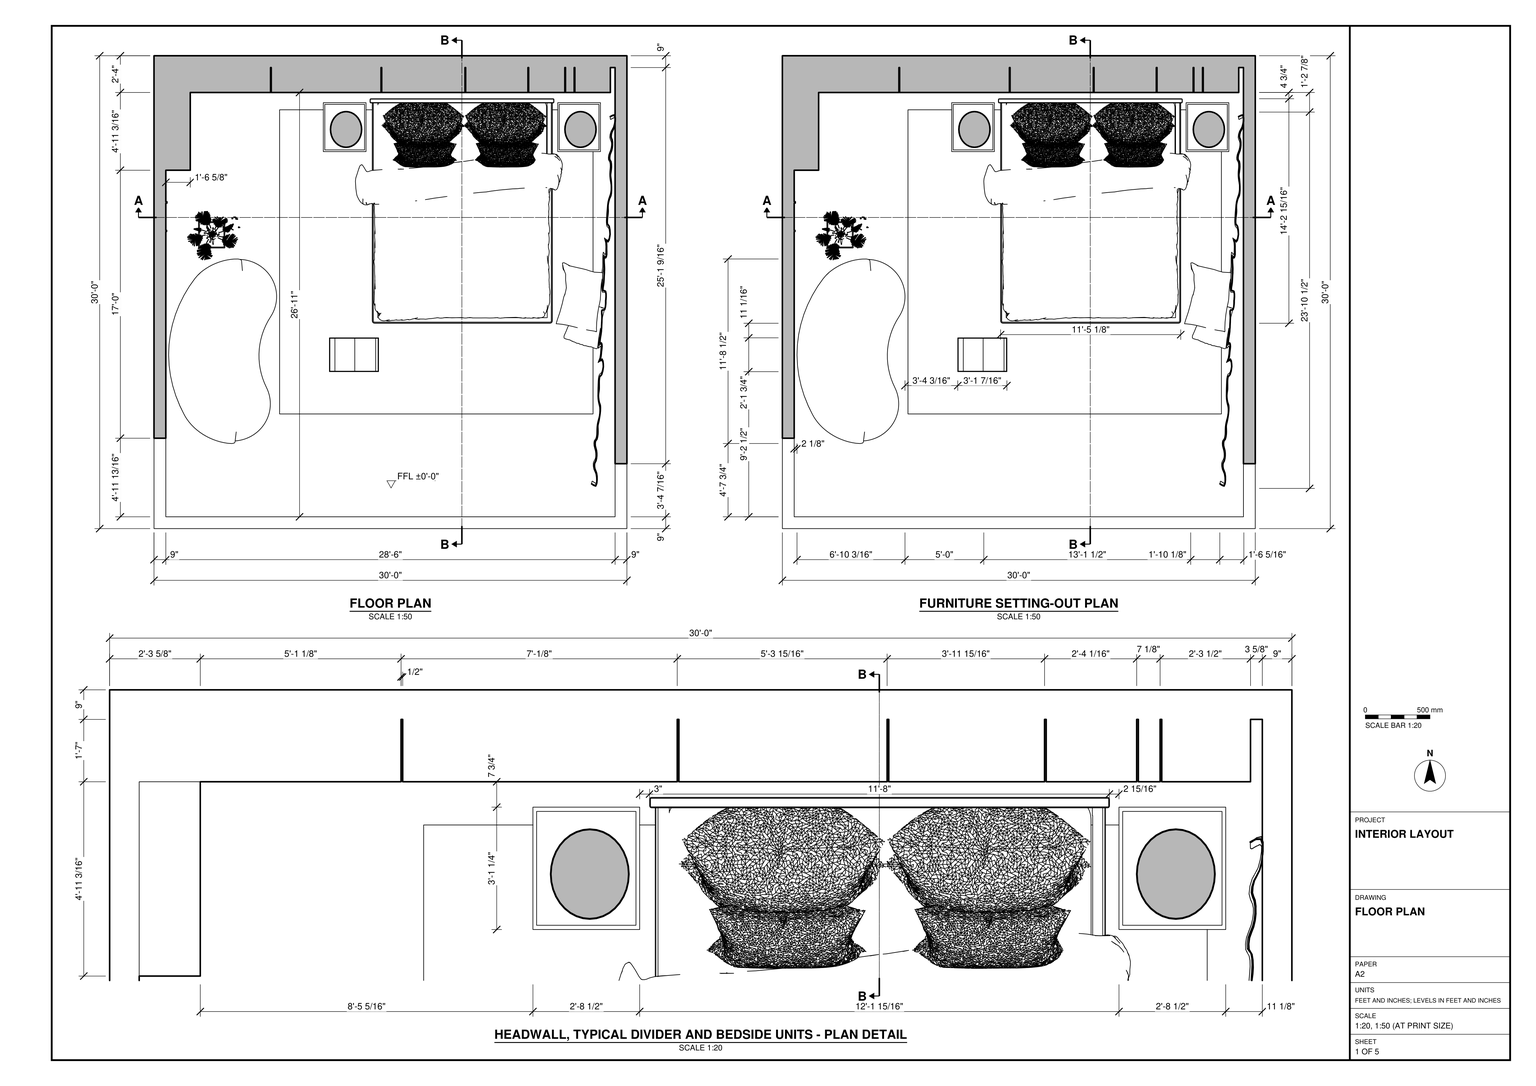
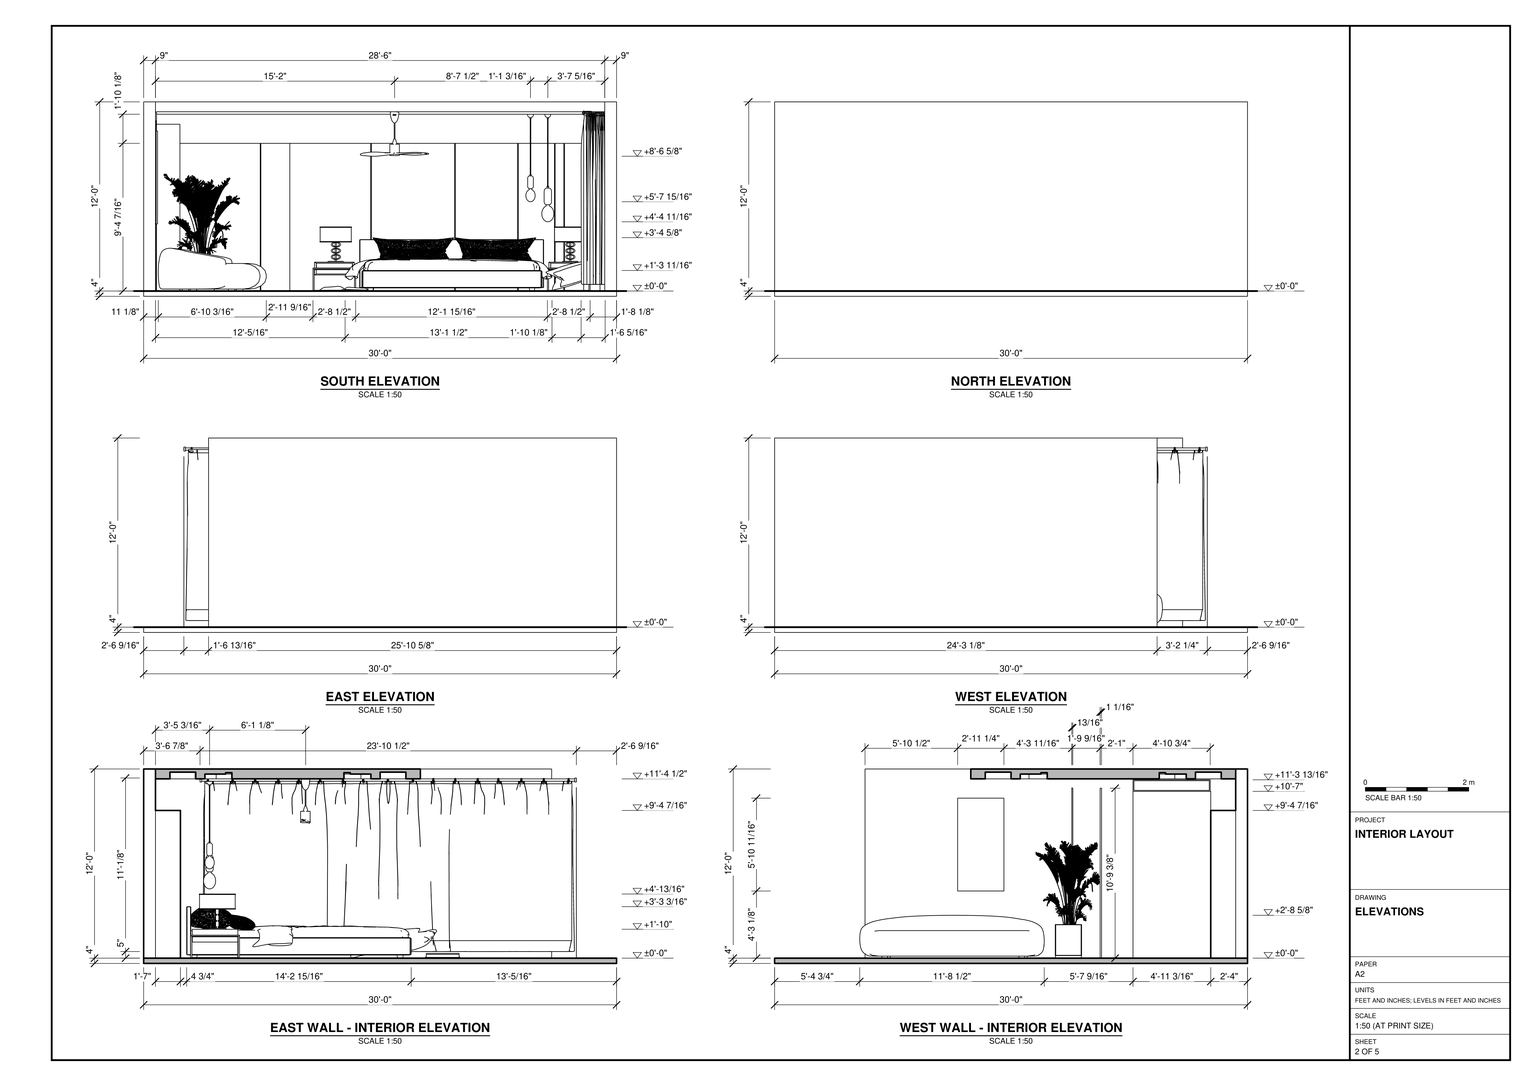
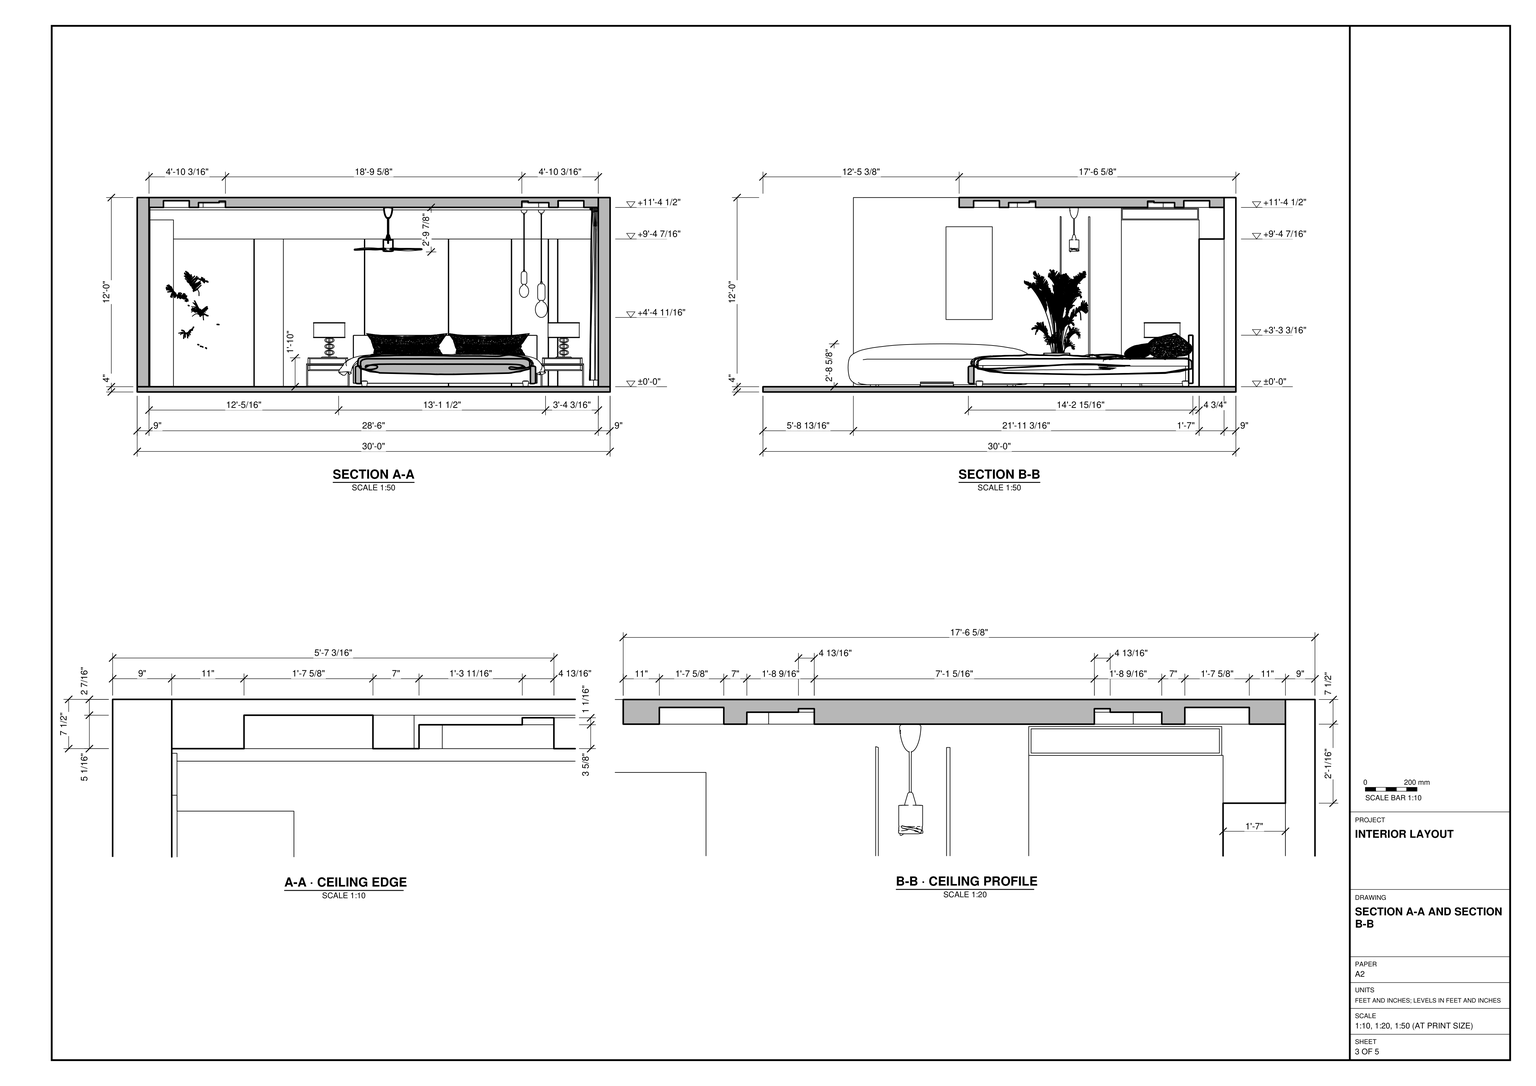
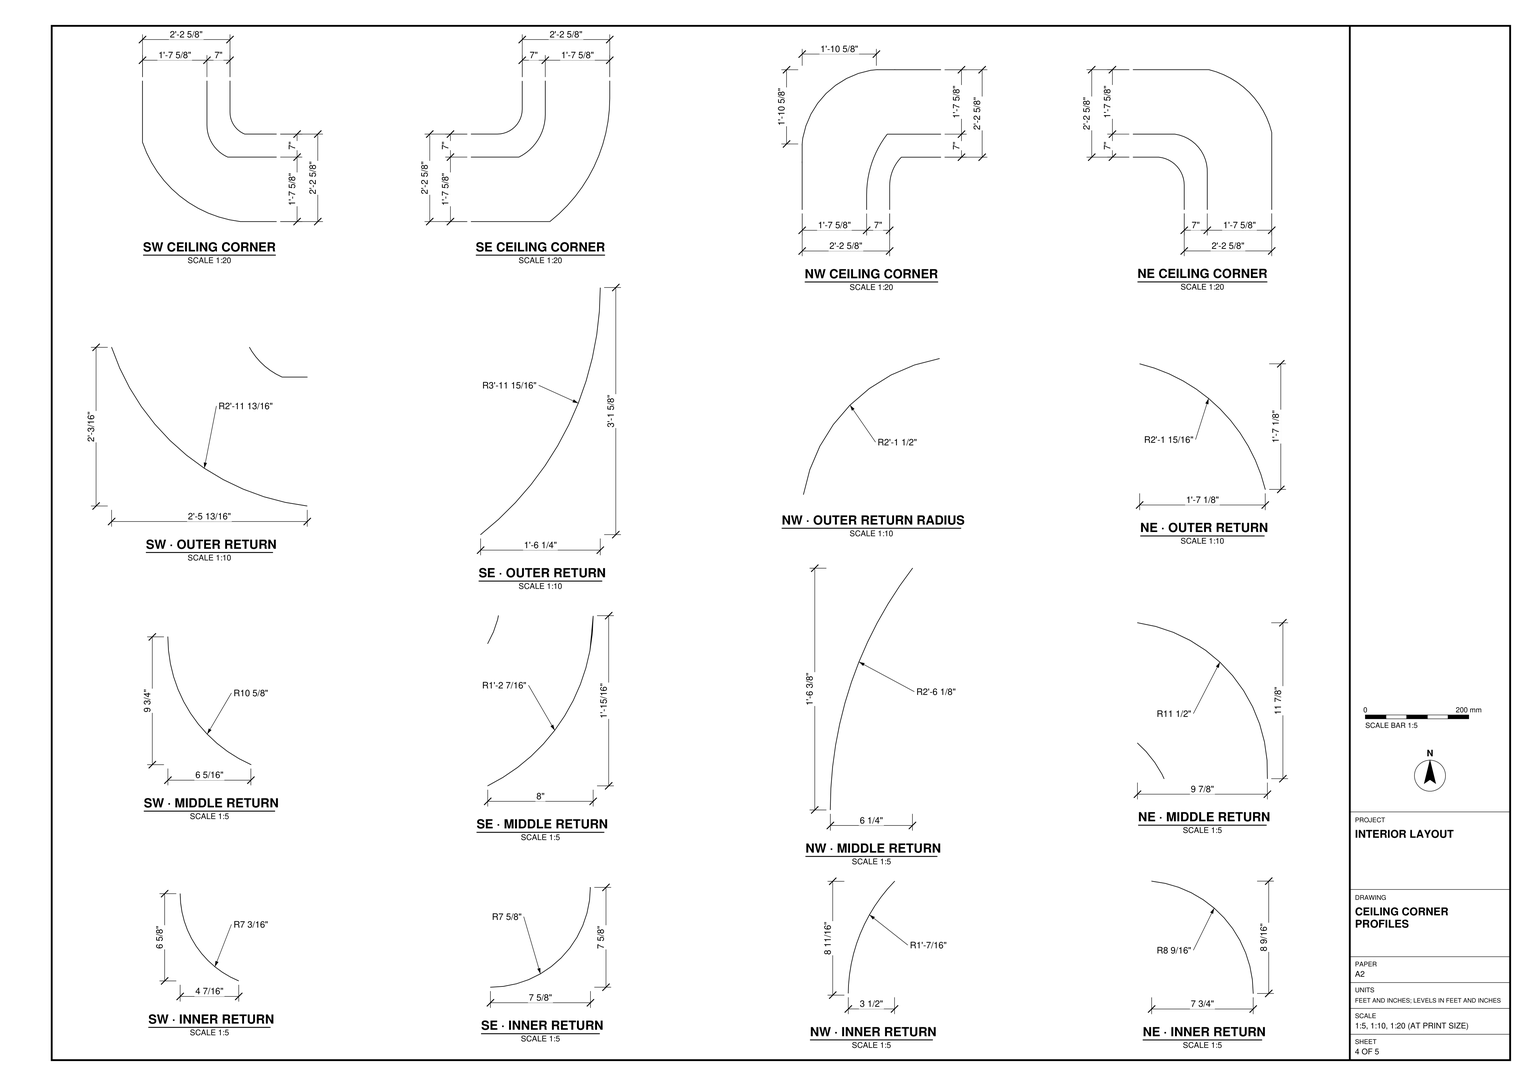
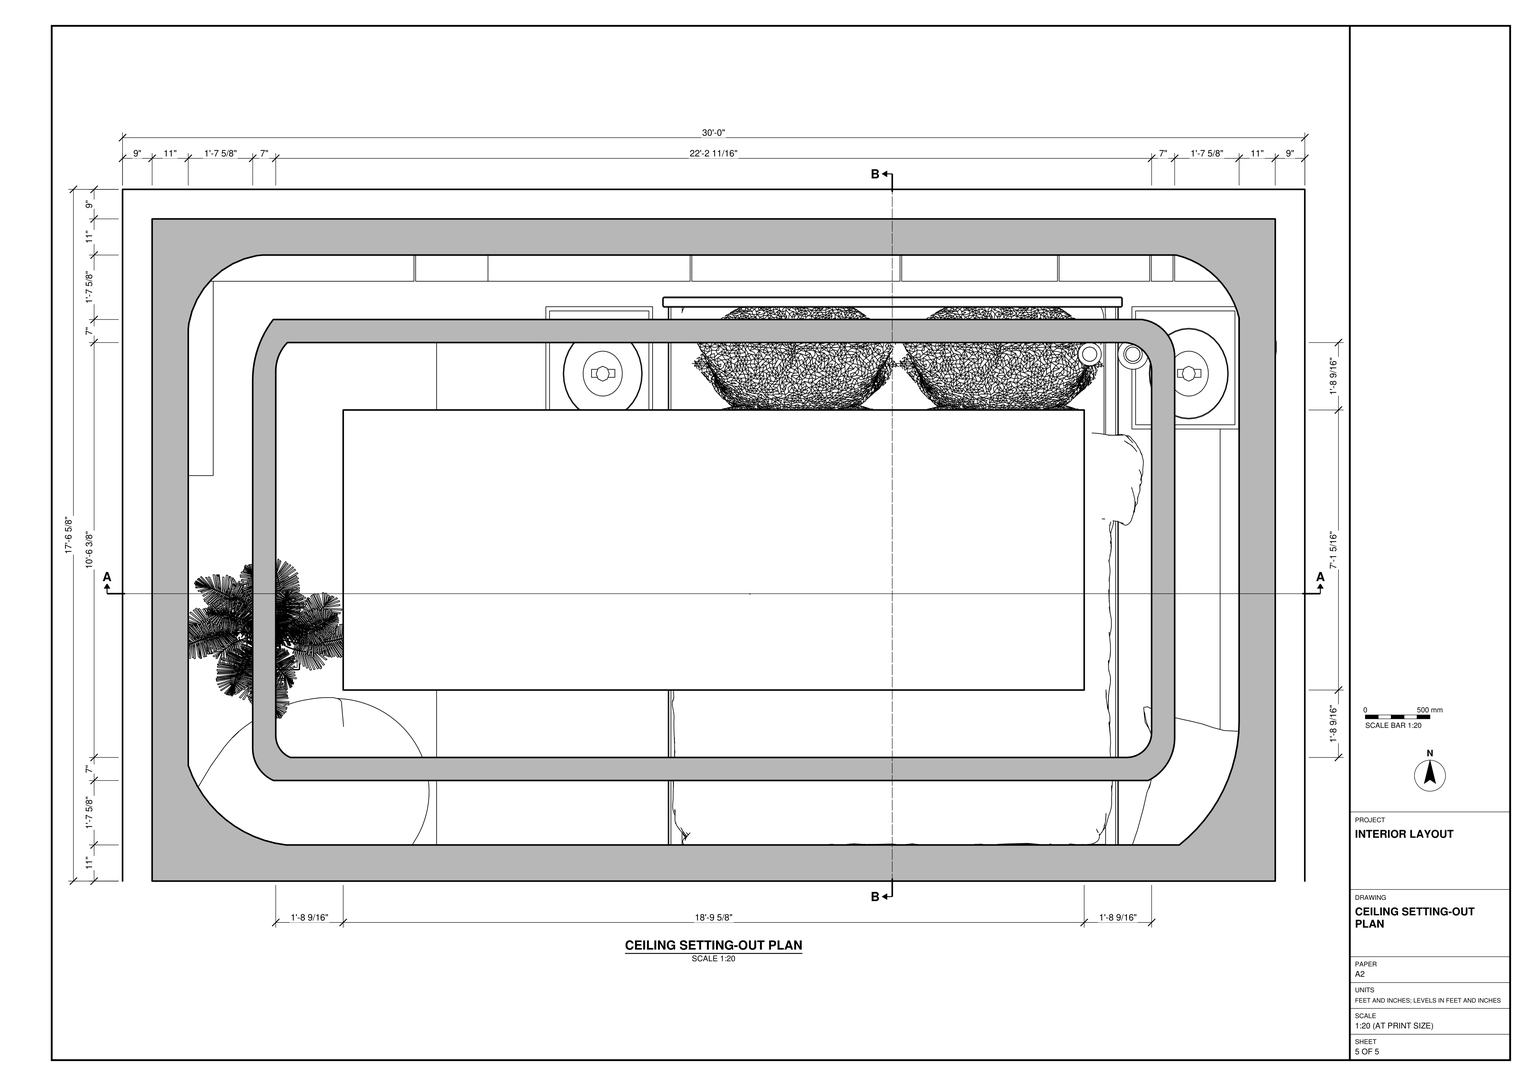
Build the bedroom interior in SketchUp from task_files/diagram_01.pdf. Work in feet and inches. The model is 30'-0" wide by 30'-0" deep and 12'-4" high overall, with one finished floor level at ±0'-0". Use the top of the 4" floor slab as the finished floor. Model the 9" walls along the north, east and west sides. Keep the south side open and stop each side wall where the floor plan shows it.

Build the headwall along the north wall, including its return, vertical panel divisions and the horizontal section above the panels. Use the sections and enlarged ceiling details to form the stepped recesses over the bed. Place the bed toward the east side of the headwall, with its foot facing south and a bedside unit on either side. Use the furniture setting-out plan for the bed footprint and the position of the curved sofa along the west side. Include the curtain along the east side, the ceiling fan, the lights and the plant in their drawn positions. Decor and loose items may be any suitable library components.

Keep the slab, walls and ceiling as separate groups or components. Do the same for each furniture or joinery piece, and use components for repeated parts. Save one SketchUp model as output_files/bedroom_with_panelled_headwall_and_stepped_ceiling.skp.

# SketchUp Ruby script. Lengths in inches.
U = 1.inch
M = Sketchup.active_model
def pt(a) = Geom::Point3d.new(a.map { |v| v * U })
def face(e, loops, mat)
  f = e.add_face(loops[0].map { |a| pt(a) })
  loops[1..].each { |l| e.add_face(l.map { |a| pt(a) }).erase! }
  f.material = f.back_material = mat if mat
  f
end
# faces: each face lists its corners as indices into pts; further lists are holes
def faces(e, pts, list, mat = nil) = list.each { |f| face(e, (f[0].is_a?(Array) ? f : [f]).map { |l| l.map { |i| pts[i] } }, mat) }
# xy, xz, yz: faces in a plane at the given z, y or x. An outline is a flat list of corners, or four numbers for a rectangle; further outlines are holes
def ring(l) = l.size == 4 ? [[l[0], l[1]], [l[2], l[1]], [l[2], l[3]], [l[0], l[3]]] : l.each_slice(2).to_a
def flat(e, list, mat, &to3) = list.each { |f| face(e, (f[0].is_a?(Array) ? f : [f]).map { |l| ring(l).map { |u, v| to3.(u, v) } }, mat) }
def xy(e, z, list, mat = nil) = flat(e, list, mat) { |x, y| [x, y, z] }
def xz(e, y, list, mat = nil) = flat(e, list, mat) { |x, z| [x, y, z] }
def yz(e, x, list, mat = nil) = flat(e, list, mat) { |y, z| [x, y, z] }
def lines(e, pts, list) = list.each { |a, b| e.add_line(pt(pts[a]), pt(pts[b])) }
# prism: a flat outline (further loops are holes) pulled along v
def prism(e, loops, v, mat = nil)
  f = face(e, loops, mat); d = Geom::Vector3d.new(v.map { |x| x * U })
  f.pushpull(f.normal.samedirection?(d) ? d.length : -d.length)
end
def box(e, o, s, mat = nil) = prism(e, [[o, [o[0] + s[0], o[1], o[2]], [o[0] + s[0], o[1] + s[1], o[2]], [o[0], o[1] + s[1], o[2]]]], [0, 0, s[2]], mat)
def at(x, y, z, deg = 0) = Geom::Transformation.translation(pt([x, y, z])) * Geom::Transformation.rotation(ORIGIN, Z_AXIS, deg.degrees)
def axes(o, x, y, z) = Geom::Transformation.new([*x, 0, *y, 0, *z, 0, *pt(o).to_a, 1])
def part(name) = M.definitions.add(name)
# library, detail: a bought-in or finely detailed component or shape, given as its bounding box
def library(name, o, s) = part(name).tap { |d| box(d.entities, o, s) }
def detail(e, o, s) = box(e.add_group.entities, o, s)
def put(e, d, t, mat = nil) = e.add_instance(d, t).tap { |i| i.material = mat if mat }
def group(e, t, mat = nil) = e.add_group.tap { |g| g.transformation = t; g.material = mat if mat }.entities
root = M.entities
M.materials.add("767e70173236cc395a06543cd97f68ed").color = [135, 135, 103]
M.materials.add("Brick_05_1K").color = [195, 185, 161]
M.materials.add("Brick_09_1K").color = [135, 129, 110]
M.materials.add("Emissive").color = [152, 121, 26]
M.materials["Emissive"].alpha = 0.92
M.materials.add("Generic").color = [255, 255, 255]
M.materials.add("M03_Pewter_Shine").color = [168, 168, 168]
M.materials.add("M05_Graphite_Haze").color = [114, 114, 114]
M.materials.add("M09_Shadow_Night").color = [0, 0, 0]
M.materials.add("Marble_01_1K").color = [230, 221, 211]
M.materials.add("Marble_06_1K").color = [165, 150, 147]
M.materials.add("Plywood_01_1K").color = [125, 96, 64]
M.materials.add("Roofing_02_1K").color = [97, 118, 74]
M.materials.add("Wicker_07_1K").color = [113, 105, 85]
M.materials.add("[0137_Black]").color = [0, 0, 0]
c1 = library("Bed_white",[-15.5625,-0.07,0],[116.82,82.58,48.83])
c2 = library("01_FANZART_BLAZE",[-27.75,-0.47,-4.86],[52.01,7.42,18.04])
c3 = library("BCL - 290",[0,0,0],[78.74,35.43,27.56])
c4 = library("flowers vase",[-18.85,-34.71,0],[57.98,48.66,89.2])
c5 = library("Pillow pair",[0,0,0],[18.27,24.9,18.7])
c6 = library("Open book",[0,0,0],[17.5,14.74,1.7])
c7 = part("fantasy")
g1 = group(c7.entities,at(-0.1875,90,-18))
xy(g1,0,[[0.75,-24,1.75,0]],"[0137_Black]")
xy(g1,53.34,[[0.75,-24,1.75,0]],"[0137_Black]")
xz(g1,-24,[[0.75,0,1.75,53.34]],"[0137_Black]")
xz(g1,0,[[0.75,0,1.75,53.34]],"[0137_Black]")
yz(g1,0.75,[[-24,0,0,53.34]])
yz(g1,1.75,[[-24,0,0,53.34]],"767e70173236cc395a06543cd97f68ed")
p = [[0,-72,137.16],[0.75,-72,137.16],[0,0,137.16],[0.75,0,137.16],[0,-72,0],[0.75,-72,0],
  [0,0,0],[0.75,0,0]]
lines(g1,p,[[0,1],[2,3],[4,5],[6,7]])
c8 = library("LIGHT",[18.68,10.22,-4.92],[21.31,9.19,61.7])
c9 = library("SHOWER+CURTAIN",[0,-2.58,0],[59,4.99,76.02])
c10 = library("Spot Light\#1",[-5.1,-5.1,-11.05],[10.2,10.2,11.05])
xy(root,4,[[0,0,360,0,360,49.41,351,49.41,351,9,9,9,9,68.83,0,68.83]])
xy(root,4,[[9,247.8125,9.81,248.88]],"Generic")
xy(root,4,[[9,272.84,27.6,332.01]],"Marble_01_1K")
xy(root,116.4375,[[347.1,332.01,347.4,351]])
xy(root,116.4375,[[111.27,332.01,172.84,351]],"M03_Pewter_Shine")
xy(root,116.4375,[[9,332.01,88.74,351],[89.24,332.01,111.27,351],[173.34,332.01,236.74,351],[237.24,332.01,284.69,351],[285.19,332.01,312.74,351],
  [313.24,332.01,319.875,351],[320.375,332.01,347.1,351]],"Marble_01_1K")
xy(root,130.98,[[9.8,272.84,27.6,272.84,27.6,332.01,9,332.01,9,331.61,9.8,331.61]],"Marble_01_1K")
xy(root,131.7,[[9,273.55,9.8,330.89]],"Generic")
xy(root,133.4,[[9,247.8125,9.81,248.88]],"Generic")
xy(root,139.08,[[9,273.55,9.8,330.89]],"Generic")
xy(root,139.79,[[9,272.84,9.8,331.61]],"Generic")
xy(root,140.5,[[20,311.39,19.79,315.27,20,317.4],[42.6,340,44.73,340.21,48.61,340]])
xy(root,140.5,[[67.18,207.54,292.82,292.82]],"M03_Pewter_Shine")
xy(root,140.5,[[[9,149.35,351,351],[49.81,160.35,321.77,160.35,324.51,162.69,327.07,165.23,329.43,167.95,331.58,170.85,333.51,173.89,335.2,177.07,336.65,180.375,337.85,183.77,338.78,187.25,339.46,190.79,339.86,194.375,340,197.97,340,320.85,339.34,323.13,338.47,325.34,337.41,327.46,336.15,329.47,334.72,331.37,333.12,333.12,331.37,334.72,329.47,336.15,327.46,337.41,325.34,338.47,323.13,339.34,320.85,340,48.61,340,44.73,340.21,42.6,340,40.86,339.83,37.09,338.86,33.51,337.33,30.21,335.28,27.26,332.74,24.72,329.79,22.67,326.49,21.14,322.91,20.17,319.14,20,317.4,19.79,315.27,20,311.39,20,184.51,21.23,181.37,22.74,178.36,24.53,175.5,26.58,172.82,28.88,170.35,31.39,168.1,34.11,166.1,37.01,164.37,40.05,162.92,43.22,161.76,46.48,160.9]],[[45.96,179.99,45.05,180.44,44.18,180.98,43.375,181.61,42.63,182.31,41.95,183.07,41.35,183.9,40.84,184.78,40.41,185.71,40.07,186.67,39.83,187.67,39.68,188.68,39.63,189.7,39.63,301.98,39.68,303.625,39.8125,305.27,40.04,306.9,40.35,308.52,40.75,310.12,41.24,311.69,41.8125,313.24,42.47,314.75,43.21,316.22,44.03,317.65,44.92,319.04,45.89,320.37,310.49,320.37,311.87,320.09,313.21,319.64,314.48,319.03,315.67,318.27,316.76,317.37,317.72,316.34,318.56,315.2,319.25,313.97,319.78,312.66,320.15,311.3,320.34,309.9,320.37,308.49,320.37,192.93,320.31,191.6,320.12,190.27,319.8125,188.97,319.39,187.7,318.85,186.48,318.2,185.3125,317.44,184.21,316.58,183.18,315.64,182.24,314.61,181.39,313.5,180.63,312.34,179.99],[51.11,187,305.74,187,306.74,187.07,307.71,187.26,308.66,187.58,309.55,188.02,310.375,188.57,311.125,189.23,311.78,189.98,312.33,190.8,312.77,191.7,313.09,192.64,313.29,193.62,313.35,194.61,313.35,304.8,313.29,305.85,313.09,306.89,312.78,307.89,312.34,308.85,311.79,309.74,311.13,310.57,310.38,311.3,309.54,311.9375,308.64,312.47,307.67,312.89,306.66,313.18,305.62,313.35,50.1875,313.35,49.65,312.76,49.14,312.13,48.68,311.48,48.27,310.79,47.89,310.08,47.57,309.35,47.29,308.6,47.06,307.83,46.88,307.05,46.75,306.26,46.67,305.46,46.65,304.66,46.65,193.65,46.68,192.94,46.79,192.24,46.96,191.55,47.2,190.89,47.5,190.25,47.87,189.64,48.29,189.08,48.77,188.55,49.29,188.08,49.86,187.66,50.47,187.3]]],"Roofing_02_1K")
xy(root,144.13,[[[51.11,187,50.47,187.3,49.86,187.66,49.29,188.08,48.77,188.55,48.29,189.08,47.87,189.64,47.5,190.25,47.2,190.89,46.96,191.55,46.79,192.24,46.68,192.94,46.65,193.65,46.65,304.66,46.67,305.46,46.75,306.26,46.88,307.05,47.06,307.83,47.29,308.6,47.57,309.35,47.89,310.08,48.27,310.79,48.68,311.48,49.14,312.13,49.65,312.76,50.1875,313.35,305.62,313.35,306.66,313.18,307.67,312.89,308.64,312.47,309.54,311.9375,310.38,311.3,311.13,310.57,311.79,309.74,312.34,308.85,312.78,307.89,313.09,306.89,313.29,305.85,313.35,304.8,313.35,194.61,313.29,193.62,313.09,192.64,312.77,191.7,312.33,190.8,311.78,189.98,311.125,189.23,310.375,188.57,309.55,188.02,308.66,187.58,307.71,187.26,306.74,187.07,305.74,187],[62.37,202.72,297.63,297.63]]],"M03_Pewter_Shine")
xy(root,145.2,[[[62.37,202.72,297.63,297.63],[67.18,207.54,292.82,292.82]]],"M09_Shadow_Night")
xy(root,145.59,[[[49.81,160.35,46.48,160.9,43.22,161.76,40.05,162.92,37.01,164.37,34.11,166.1,31.39,168.1,28.88,170.35,26.58,172.82,24.53,175.5,22.74,178.36,21.23,181.37,20,184.51,20,317.4,20.17,319.14,21.14,322.91,22.67,326.49,24.72,329.79,27.26,332.74,30.21,335.28,33.51,337.33,37.09,338.86,40.86,339.83,42.6,340,320.85,340,323.13,339.34,325.34,338.47,327.46,337.41,329.47,336.15,331.37,334.72,333.12,333.12,334.72,331.37,336.15,329.47,337.41,327.46,338.47,325.34,339.34,323.13,340,320.85,340,197.97,339.86,194.375,339.46,190.79,338.78,187.25,337.85,183.77,336.65,180.375,335.2,177.07,333.51,173.89,331.58,170.85,329.43,167.95,327.07,165.23,324.51,162.69,321.77,160.35],[45.96,179.99,312.34,179.99,313.5,180.63,314.61,181.39,315.64,182.24,316.58,183.18,317.44,184.21,318.2,185.3125,318.85,186.48,319.39,187.7,319.8125,188.97,320.12,190.27,320.31,191.6,320.37,192.93,320.37,308.49,320.34,309.9,320.15,311.3,319.78,312.66,319.25,313.97,318.56,315.2,317.72,316.34,316.76,317.37,315.67,318.27,314.48,319.03,313.21,319.64,311.87,320.09,310.49,320.37,45.89,320.37,44.92,319.04,44.03,317.65,43.21,316.22,42.47,314.75,41.8125,313.24,41.24,311.69,40.75,310.12,40.35,308.52,40.04,306.9,39.8125,305.27,39.68,303.625,39.63,301.98,39.63,189.7,39.68,188.68,39.83,187.67,40.07,186.67,40.41,185.71,40.84,184.78,41.35,183.9,41.95,183.07,42.63,182.31,43.375,181.61,44.18,180.98,45.05,180.44]]],"M03_Pewter_Shine")
xy(root,148,[[351,49.41,360,149.35],[0,68.83,9,149.35],[0,149.35,9,149.35,9,351,351,351,351,149.35,360,149.35,360,360,0,360],[9,149.35,351,351]])
xz(root,49.41,[[351,4,360,148]])
xz(root,68.83,[[0,4,9,148]])
xz(root,149.35,[[9,140.5,351,148]])
xz(root,160.35,[[49.81,140.5,321.77,145.59]],"Emissive")
xz(root,179.99,[[45.96,140.5,312.34,145.59]],"Roofing_02_1K")
xz(root,187,[[51.11,140.5,305.74,144.13]],"Emissive")
xz(root,202.72,[[62.37,144.13,297.63,145.2]])
xz(root,207.54,[[67.18,140.5,292.82,145.2]],"Emissive")
xz(root,226.23,[[9,4.27,9.5625,133.67]],"Wicker_07_1K")
xz(root,227.03,[[9,4,9.5625,133.4]],"M05_Graphite_Haze")
xz(root,247.8125,[[9,4,9.81,133.4]],"Wicker_07_1K")
xz(root,248.88,[[9,4,9.81,133.4]],"Generic")
xz(root,272.84,[[9,4,27.6,130.98]],"Marble_01_1K")
xz(root,272.84,[[9,130.98,9.8,139.79]],"Wicker_07_1K")
xz(root,273.55,[[9,131.7,9.8,139.08]],"Generic")
xz(root,292.82,[[67.18,140.5,292.82,145.2]],"Emissive")
xz(root,297.63,[[62.37,144.13,297.63,145.2]],"M09_Shadow_Night")
xz(root,313.35,[[50.1875,140.5,305.62,144.13]],"Emissive")
xz(root,320.37,[[45.89,140.5,310.49,145.59]])
xz(root,330.89,[[9,131.7,9.8,139.08]],"Wicker_07_1K")
xz(root,331.61,[[9,130.98,9.8,139.79]],"Generic")
xz(root,332.01,[[27.6,4,88.74,116.4375],[89.24,4,111.27,116.4375],[173.34,4,236.74,116.4375],[237.24,4,284.69,116.4375],[285.19,4,312.74,116.4375],
  [313.24,4,319.875,116.4375],[320.375,4,347.4,116.4375],[9,116.4375,27.6,130.98]],"Marble_01_1K")
xz(root,332.01,[[111.27,4,172.84,116.4375]],"Marble_06_1K")
xz(root,340,[[42.6,140.5,48.61,145.59],[48.61,140.5,320.85,145.59]],"Emissive")
xz(root,351,[[347.4,4,351,4,351,140.5,9,140.5,9,138.59,347.1,138.59,347.1,116.4375,347.4,116.4375],[88.74,4,89.24,116.4375],[172.84,4,173.34,116.4375],[236.74,4,237.24,116.4375],[284.69,4,285.19,116.4375],
  [312.74,4,313.24,116.4375],[319.875,4,320.375,116.4375],[9,140.5,351,148]])
xz(root,351,[[9,116.4375,347.1,138.59]],"Plywood_01_1K")
xz(root,360,[[0,4,360,148]])
yz(root,0,[[68.83,4,360,148]])
yz(root,9,[[149.35,140.5,351,148]])
yz(root,9,[[68.83,4,145.9375,4,226.23,4.27,226.23,133.67,227.03,133.4,227.03,4,247.8125,4,247.8125,133.4,248.88,133.4,248.88,4,272.84,4,272.84,139.79,331.61,139.79,331.61,130.98,332.01,130.98,332.01,116.4375,351,116.4375,351,140.5,149.35,140.5,149.35,148,68.83,148]],"M05_Graphite_Haze")
yz(root,9,[[273.55,131.7,330.89,139.08]],"Wicker_07_1K")
yz(root,9.5625,[[227.03,4,227.03,133.4,226.23,133.67,226.23,4.27]],"Wicker_07_1K")
yz(root,9.8,[[[272.84,130.98,331.61,139.79],[273.55,131.7,330.89,139.08]]],"Wicker_07_1K")
yz(root,9.81,[[247.8125,4,248.88,133.4]],"Wicker_07_1K")
yz(root,20,[[184.51,140.5,311.39,145.59],[311.39,140.5,317.4,145.59]],"Emissive")
yz(root,27.6,[[272.84,4,332.01,130.98]],"Marble_01_1K")
yz(root,39.63,[[189.7,140.5,301.98,145.59]])
yz(root,46.65,[[193.65,140.5,304.66,144.13]],"Emissive")
yz(root,62.37,[[202.72,144.13,297.63,145.2]],"M09_Shadow_Night")
yz(root,67.18,[[207.54,140.5,292.82,145.2]],"Emissive")
yz(root,88.74,[[332.01,4,351,116.4375]])
yz(root,89.24,[[332.01,4,351,116.4375]])
yz(root,172.84,[[332.01,4,351,116.4375]])
yz(root,173.34,[[332.01,4,351,116.4375]])
yz(root,236.74,[[332.01,4,351,116.4375]])
yz(root,237.24,[[332.01,4,351,116.4375]])
yz(root,284.69,[[332.01,4,351,116.4375]])
yz(root,285.19,[[332.01,4,351,116.4375]])
yz(root,292.82,[[207.54,140.5,292.82,145.2]],"Emissive")
yz(root,297.63,[[202.72,144.13,297.63,145.2]])
yz(root,312.74,[[332.01,4,351,116.4375]])
yz(root,313.24,[[332.01,4,351,116.4375]])
yz(root,313.35,[[194.61,140.5,304.8,144.13]],"Emissive")
yz(root,319.875,[[332.01,4,351,116.4375]])
yz(root,320.37,[[192.93,140.5,308.49,145.59]])
yz(root,320.375,[[332.01,4,351,116.4375]])
yz(root,340,[[197.97,140.5,320.85,145.59]],"Emissive")
yz(root,347.4,[[332.01,4,351,116.4375]])
yz(root,351,[[149.35,140.5,351,148]])
yz(root,351,[[49.41,4,49.41,148,149.35,148,149.35,140.5,351,140.5,351,4]],"Generic")
yz(root,360,[[49.41,4,360,148]])
p = [[9,226.23,4.27],[9,227.03,4],[9.5625,227.03,4],[9.5625,226.23,4.27],[9,227.03,133.4],[9,226.23,133.67],
  [9.5625,226.23,133.67],[9.5625,227.03,133.4],[49.81,160.35,140.5],[46.48,160.9,140.5],[46.48,160.9,145.59],[49.81,160.35,145.59],
  [324.51,162.69,140.5],[321.77,160.35,140.5],[321.77,160.35,145.59],[324.51,162.69,145.59],[43.22,161.76,140.5],[43.22,161.76,145.59],
  [40.05,162.92,140.5],[40.05,162.92,145.59],[327.07,165.23,140.5],[327.07,165.23,145.59],[37.01,164.37,140.5],[37.01,164.37,145.59],
  [34.11,166.1,140.5],[34.11,166.1,145.59],[329.43,167.95,140.5],[329.43,167.95,145.59],[31.39,168.1,140.5],[31.39,168.1,145.59],
  [331.58,170.85,140.5],[331.58,170.85,145.59],[28.88,170.35,140.5],[28.88,170.35,145.59],[26.58,172.82,140.5],[26.58,172.82,145.59],
  [333.51,173.89,140.5],[333.51,173.89,145.59],[24.53,175.5,140.5],[24.53,175.5,145.59],[335.2,177.07,140.5],[335.2,177.07,145.59],
  [22.74,178.36,140.5],[22.74,178.36,145.59],[336.65,180.375,140.5],[336.65,180.375,145.59],[21.23,181.37,140.5],[21.23,181.37,145.59],
  [45.05,180.44,140.5],[45.96,179.99,140.5],[45.96,179.99,145.59],[45.05,180.44,145.59],[312.34,179.99,140.5],[313.5,180.63,140.5],
  [313.5,180.63,145.59],[312.34,179.99,145.59],[44.18,180.98,140.5],[44.18,180.98,145.59],[337.85,183.77,140.5],[337.85,183.77,145.59],
  [314.61,181.39,140.5],[314.61,181.39,145.59],[43.375,181.61,140.5],[43.375,181.61,145.59],[20,184.51,140.5],[20,184.51,145.59],
  [315.64,182.24,140.5],[315.64,182.24,145.59],[42.63,182.31,140.5],[42.63,182.31,145.59],[316.58,183.18,140.5],[316.58,183.18,145.59],
  [41.95,183.07,140.5],[41.95,183.07,145.59],[41.35,183.9,140.5],[41.35,183.9,145.59],[317.44,184.21,140.5],[317.44,184.21,145.59],
  [338.78,187.25,140.5],[338.78,187.25,145.59],[40.84,184.78,140.5],[40.84,184.78,145.59],[318.2,185.3125,140.5],[318.2,185.3125,145.59],
  [40.41,185.71,140.5],[40.41,185.71,145.59],[318.85,186.48,140.5],[318.85,186.48,145.59],[40.07,186.67,140.5],[40.07,186.67,145.59],
  [319.39,187.7,140.5],[319.39,187.7,145.59],[39.83,187.67,140.5],[39.83,187.67,145.59],[51.11,187,140.5],[50.47,187.3,140.5],
  [50.47,187.3,144.13],[51.11,187,144.13],[306.74,187.07,140.5],[305.74,187,140.5],[305.74,187,144.13],[306.74,187.07,144.13],
  [307.71,187.26,140.5],[307.71,187.26,144.13],[49.86,187.66,140.5],[49.86,187.66,144.13],[308.66,187.58,140.5],[308.66,187.58,144.13],
  [339.46,190.79,140.5],[339.46,190.79,145.59],[309.55,188.02,140.5],[309.55,188.02,144.13],[39.68,188.68,140.5],[39.68,188.68,145.59],
  [49.29,188.08,140.5],[49.29,188.08,144.13],[319.8125,188.97,140.5],[319.8125,188.97,145.59],[310.375,188.57,140.5],[310.375,188.57,144.13],
  [48.77,188.55,140.5],[48.77,188.55,144.13],[48.29,189.08,140.5],[48.29,189.08,144.13],[311.125,189.23,140.5],[311.125,189.23,144.13],
  [39.63,189.7,140.5],[39.63,189.7,145.59],[320.12,190.27,140.5],[320.12,190.27,145.59],[47.87,189.64,140.5],[47.87,189.64,144.13],
  [311.78,189.98,140.5],[311.78,189.98,144.13],[47.5,190.25,140.5],[47.5,190.25,144.13],[312.33,190.8,140.5],[312.33,190.8,144.13],
  [47.2,190.89,140.5],[47.2,190.89,144.13],[320.31,191.6,140.5],[320.31,191.6,145.59],[312.77,191.7,140.5],[312.77,191.7,144.13],
  [339.86,194.375,140.5],[339.86,194.375,145.59],[46.96,191.55,140.5],[46.96,191.55,144.13],[46.79,192.24,140.5],[46.79,192.24,144.13],
  [320.37,192.93,140.5],[320.37,192.93,145.59],[313.09,192.64,140.5],[313.09,192.64,144.13],[46.68,192.94,140.5],[46.68,192.94,144.13],
  [313.29,193.62,140.5],[313.29,193.62,144.13],[46.65,193.65,140.5],[46.65,193.65,144.13],[313.35,194.61,140.5],[313.35,194.61,144.13],
  [340,197.97,140.5],[340,197.97,145.59],[39.68,303.625,140.5],[39.63,301.98,140.5],[39.63,301.98,145.59],[39.68,303.625,145.59],
  [39.8125,305.27,140.5],[39.8125,305.27,145.59],[46.65,304.66,140.5],[46.67,305.46,140.5],[46.67,305.46,144.13],[46.65,304.66,144.13],
  [313.29,305.85,140.5],[313.35,304.8,140.5],[313.35,304.8,144.13],[313.29,305.85,144.13],[40.04,306.9,140.5],[40.04,306.9,145.59],
  [46.75,306.26,140.5],[46.75,306.26,144.13],[313.09,306.89,140.5],[313.09,306.89,144.13],[46.88,307.05,140.5],[46.88,307.05,144.13],
  [40.35,308.52,140.5],[40.35,308.52,145.59],[312.78,307.89,140.5],[312.78,307.89,144.13],[47.06,307.83,140.5],[47.06,307.83,144.13],
  [47.29,308.6,140.5],[47.29,308.6,144.13],[312.34,308.85,140.5],[312.34,308.85,144.13],[40.75,310.12,140.5],[40.75,310.12,145.59],
  [320.37,308.49,140.5],[320.34,309.9,140.5],[320.34,309.9,145.59],[320.37,308.49,145.59],[47.57,309.35,140.5],[47.57,309.35,144.13],
  [311.79,309.74,140.5],[311.79,309.74,144.13],[47.89,310.08,140.5],[47.89,310.08,144.13],[311.13,310.57,140.5],[311.13,310.57,144.13],
  [320.15,311.3,140.5],[320.15,311.3,145.59],[41.24,311.69,140.5],[41.24,311.69,145.59],[48.27,310.79,140.5],[48.27,310.79,144.13],
  [310.38,311.3,140.5],[310.38,311.3,144.13],[48.68,311.48,140.5],[48.68,311.48,144.13],[309.54,311.9375,140.5],[309.54,311.9375,144.13],
  [319.78,312.66,140.5],[319.78,312.66,145.59],[49.14,312.13,140.5],[49.14,312.13,144.13],[41.8125,313.24,140.5],[41.8125,313.24,145.59],
  [308.64,312.47,140.5],[308.64,312.47,144.13],[49.65,312.76,140.5],[49.65,312.76,144.13],[307.67,312.89,140.5],[307.67,312.89,144.13],
  [319.25,313.97,140.5],[319.25,313.97,145.59],[50.1875,313.35,140.5],[50.1875,313.35,144.13],[306.66,313.18,140.5],[306.66,313.18,144.13],
  [42.47,314.75,140.5],[42.47,314.75,145.59],[305.62,313.35,140.5],[305.62,313.35,144.13],[318.56,315.2,140.5],[318.56,315.2,145.59],
  [43.21,316.22,140.5],[43.21,316.22,145.59],[317.72,316.34,140.5],[317.72,316.34,145.59],[44.03,317.65,140.5],[44.03,317.65,145.59],
  [316.76,317.37,140.5],[316.76,317.37,145.59],[20,317.4,140.5],[20.17,319.14,140.5],[20.17,319.14,145.59],[20,317.4,145.59],
  [315.67,318.27,140.5],[315.67,318.27,145.59],[44.92,319.04,140.5],[44.92,319.04,145.59],[314.48,319.03,140.5],[314.48,319.03,145.59],
  [45.89,320.37,140.5],[45.89,320.37,145.59],[313.21,319.64,140.5],[313.21,319.64,145.59],[21.14,322.91,140.5],[21.14,322.91,145.59],
  [311.87,320.09,140.5],[311.87,320.09,145.59],[310.49,320.37,140.5],[310.49,320.37,145.59],[339.34,323.13,140.5],[340,320.85,140.5],
  [340,320.85,145.59],[339.34,323.13,145.59],[22.67,326.49,140.5],[22.67,326.49,145.59],[338.47,325.34,140.5],[338.47,325.34,145.59],
  [337.41,327.46,140.5],[337.41,327.46,145.59],[24.72,329.79,140.5],[24.72,329.79,145.59],[336.15,329.47,140.5],[336.15,329.47,145.59],
  [334.72,331.37,140.5],[334.72,331.37,145.59],[27.26,332.74,140.5],[27.26,332.74,145.59],[333.12,333.12,140.5],[333.12,333.12,145.59],
  [30.21,335.28,140.5],[30.21,335.28,145.59],[331.37,334.72,140.5],[331.37,334.72,145.59],[329.47,336.15,140.5],[329.47,336.15,145.59],
  [33.51,337.33,140.5],[33.51,337.33,145.59],[327.46,337.41,140.5],[327.46,337.41,145.59],[37.09,338.86,140.5],[37.09,338.86,145.59],
  [325.34,338.47,140.5],[325.34,338.47,145.59],[323.13,339.34,140.5],[323.13,339.34,145.59],[40.86,339.83,140.5],[40.86,339.83,145.59],
  [320.85,340,140.5],[320.85,340,145.59],[42.6,340,140.5],[42.6,340,145.59]]
faces(root,p,[[0,1,2,3],[4,5,6,7]],"Generic")
faces(root,p,[[8,9,10,11],[12,13,14,15],[9,16,17,10],[16,18,19,17],[20,12,15,21],[18,22,23,19],[22,24,25,23],[26,20,21,27],
  [24,28,29,25],[30,26,27,31],[28,32,33,29],[32,34,35,33],[36,30,31,37],[34,38,39,35],[40,36,37,41],[38,42,43,39],
  [44,40,41,45],[42,46,47,43],[58,44,45,59],[46,64,65,47],[78,58,59,79],[94,95,96,97],[98,99,100,101],[102,98,101,103],
  [95,104,105,96],[106,102,103,107],[108,78,79,109],[110,106,107,111],[104,114,115,105],[118,110,111,119],[114,120,121,115],[120,122,123,121],
  [124,118,119,125],[122,130,131,123],[132,124,125,133],[130,134,135,131],[136,132,133,137],[134,138,139,135],[142,136,137,143],[144,108,109,145],
  [138,146,147,139],[146,148,149,147],[152,142,143,153],[148,154,155,149],[156,152,153,157],[154,158,159,155],[160,156,157,161],[162,144,145,163],
  [170,171,172,173],[174,175,176,177],[171,180,181,172],[182,174,177,183],[180,184,185,181],[188,182,183,189],[184,190,191,185],[190,192,193,191],
  [194,188,189,195],[192,202,203,193],[204,194,195,205],[202,206,207,203],[208,204,205,209],[206,214,215,207],[216,208,209,217],[214,218,219,215],
  [220,216,217,221],[218,224,225,219],[228,220,221,229],[224,230,231,225],[232,228,229,233],[230,236,237,231],[238,232,233,239],[242,238,239,243],
  [254,255,256,257],[255,268,269,256],[274,275,276,277],[268,278,279,269],[280,274,277,281],[282,280,281,283],[278,284,285,279],[286,282,283,287],
  [288,286,287,289],[284,290,291,285],[292,288,289,293],[290,294,295,291],[296,292,293,297],[298,296,297,299],[294,300,301,295],[302,298,299,303],
  [300,304,305,301],[306,302,303,307],[308,306,307,309],[304,310,311,305],[312,308,309,313],[310,314,315,311]],"Emissive")
faces(root,p,[[48,49,50,51],[52,53,54,55],[56,48,51,57],[53,60,61,54],[62,56,57,63],[60,66,67,61],[68,62,63,69],[66,70,71,67],
  [72,68,69,73],[74,72,73,75],[70,76,77,71],[80,74,75,81],[76,82,83,77],[84,80,81,85],[82,86,87,83],[88,84,85,89],
  [86,90,91,87],[92,88,89,93],[112,92,93,113],[90,116,117,91],[126,112,113,127],[116,128,129,117],[128,140,141,129],[140,150,151,141]],"Roofing_02_1K")
faces(root,p,[[164,165,166,167],[168,164,167,169],[178,168,169,179],[186,178,179,187],[196,186,187,197],[198,199,200,201],[199,210,211,200],[212,196,197,213],
  [210,222,223,211],[226,212,213,227],[222,234,235,223],[240,226,227,241],[234,244,245,235],[246,240,241,247],[244,248,249,245],[250,246,247,251],
  [248,252,253,249],[252,258,259,253],[260,250,251,261],[258,262,263,259],[264,260,261,265],[262,266,267,263],[266,270,271,267],[270,272,273,271]])
put(root,c1,axes([157,156.46,4],[1.80589,0,0],[0,2.07,0],[0,0,1]))
put(root,c2,axes([192.68,233.65,115.75],[1,0,0],[0,1,0],[0,0,1.87999]))
put(root,c3,axes([86.75,63.16,4],[0.10423,1.78163,0],[-2.24471,0.13132,0],[0,0,1.1844]),"Wicker_07_1K")
put(root,c4,at(34.07,233.51,4))
put(root,c5,axes([343.2,136.97,14.68],[-0.40035,0,0.91636],[0,2.63,0],[-1.64899,0,-0.72042]))
put(root,c6,axes([133.53,119.49,4],[2.13814,0,0],[0,1.74653,0],[0,0,2.12]))
put(root,c7,axes([9,42.39,78.97],[1,0,0],[0,1.46858,0],[0,0,1.325]))
put(root,c8,axes([272.27,294.99,63.24],[1,0,0],[0,1,0],[0,0,1.32709]))
put(root,c9,axes([334.95,30.625,4],[0.24597,4.85496,0],[-0.99872,0.0506,0],[0,0,1.80412]))
put(root,c10,at(9,156.82,138.4))
put(root,c10,at(257.84,329.17,101.47))
put(root,c10,at(213.19,329.17,101.47))
g2 = group(root,at(0,0,0))
xy(g2,0,[[0,0,360,360]])
xy(g2,4,[[95.62,87.28,334.21,318.85]],"Brick_05_1K")
xy(g2,4,[[[0,0,360,360],[95.62,87.28,334.21,318.85]]],"Brick_09_1K")
xz(g2,0,[[0,0,360,4]])
xz(g2,360,[[0,0,360,4]])
yz(g2,0,[[0,0,360,4]])
yz(g2,360,[[0,0,360,4]])
